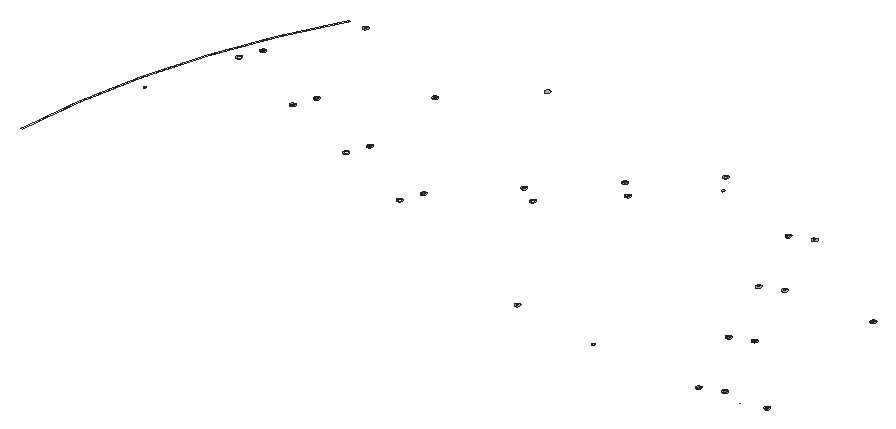
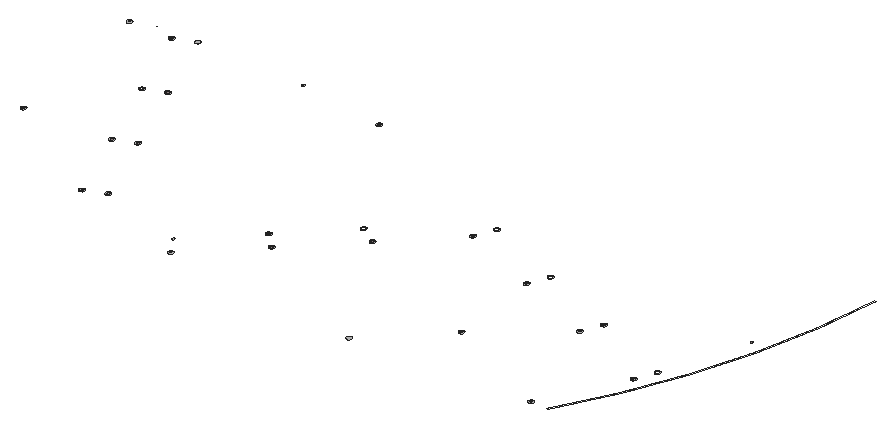
# SketchUp Ruby script. Lengths in inches.
U = 1.inch
M = Sketchup.active_model
def pt(a) = Geom::Point3d.new(a.map { |v| v * U })
def face(e, loops, mat)
  f = e.add_face(loops[0].map { |a| pt(a) })
  loops[1..].each { |l| e.add_face(l.map { |a| pt(a) }).erase! }
  f.material = f.back_material = mat if mat
  f
end
# faces: each face lists its corners as indices into pts; further lists are holes
def faces(e, pts, list, mat = nil) = list.each { |f| face(e, (f[0].is_a?(Array) ? f : [f]).map { |l| l.map { |i| pts[i] } }, mat) }
# xy, xz, yz: faces in a plane at the given z, y or x. An outline is a flat list of corners, or four numbers for a rectangle; further outlines are holes
def ring(l) = l.size == 4 ? [[l[0], l[1]], [l[2], l[1]], [l[2], l[3]], [l[0], l[3]]] : l.each_slice(2).to_a
def flat(e, list, mat, &to3) = list.each { |f| face(e, (f[0].is_a?(Array) ? f : [f]).map { |l| ring(l).map { |u, v| to3.(u, v) } }, mat) }
def xy(e, z, list, mat = nil) = flat(e, list, mat) { |x, y| [x, y, z] }
def xz(e, y, list, mat = nil) = flat(e, list, mat) { |x, z| [x, y, z] }
def yz(e, x, list, mat = nil) = flat(e, list, mat) { |y, z| [x, y, z] }
def lines(e, pts, list) = list.each { |a, b| e.add_line(pt(pts[a]), pt(pts[b])) }
# prism: a flat outline (further loops are holes) pulled along v
def prism(e, loops, v, mat = nil)
  f = face(e, loops, mat); d = Geom::Vector3d.new(v.map { |x| x * U })
  f.pushpull(f.normal.samedirection?(d) ? d.length : -d.length)
end
def box(e, o, s, mat = nil) = prism(e, [[o, [o[0] + s[0], o[1], o[2]], [o[0] + s[0], o[1] + s[1], o[2]], [o[0], o[1] + s[1], o[2]]]], [0, 0, s[2]], mat)
def at(x, y, z, deg = 0) = Geom::Transformation.translation(pt([x, y, z])) * Geom::Transformation.rotation(ORIGIN, Z_AXIS, deg.degrees)
def axes(o, x, y, z) = Geom::Transformation.new([*x, 0, *y, 0, *z, 0, *pt(o).to_a, 1])
def part(name) = M.definitions.add(name)
# library, detail: a bought-in or finely detailed component or shape, given as its bounding box
def library(name, o, s) = part(name).tap { |d| box(d.entities, o, s) }
def detail(e, o, s) = box(e.add_group.entities, o, s)
def put(e, d, t, mat = nil) = e.add_instance(d, t).tap { |i| i.material = mat if mat }
def group(e, t, mat = nil) = e.add_group.tap { |g| g.transformation = t; g.material = mat if mat }.entities
root = M.entities
M.materials.add("[Asphalt_Stamped_Brick]").color = [149, 133, 134]
M.materials.add("[Metal_Steel_Textured_White]").color = [191, 191, 191]
xy(root,3.625,[[149.02,166.314,149.015,166.316,149.011,166.32,149.008,166.324,149.006,166.329,149.005,166.334,149.006,166.339,149.008,166.344,149.011,166.348,149.015,166.351,149.02,166.353,149.025,166.354,149.031,166.353,149.035,166.351,149.04,166.348,149.043,166.344,149.045,166.339,149.045,166.329,149.043,166.324,149.04,166.32,149.035,166.316,149.031,166.314],[150.605,166.314,150.6,166.316,150.596,166.32,150.593,166.324,150.591,166.329,150.59,166.334,150.591,166.339,150.593,166.344,150.596,166.348,150.6,166.351,150.605,166.353,150.61,166.354,150.615,166.353,150.62,166.351,150.624,166.348,150.628,166.344,150.63,166.339,150.63,166.329,150.628,166.324,150.62,166.316,150.615,166.314],[141.054,166.555,141.049,166.556,141.044,166.558,141.04,166.561,141.037,166.565,141.035,166.57,141.034,166.575,141.035,166.581,141.037,166.585,141.04,166.59,141.044,166.593,141.049,166.595,141.059,166.595,141.064,166.593,141.068,166.59,141.071,166.585,141.073,166.581,141.074,166.575,141.073,166.57,141.071,166.565,141.068,166.561,141.064,166.558,141.059,166.556],[147.085,168.912,147.08,168.913,147.075,168.915,147.071,168.918,147.068,168.922,147.066,168.927,147.065,168.932,147.066,168.937,147.068,168.942,147.071,168.946,147.075,168.949,147.08,168.951,147.085,168.952,147.09,168.951,147.095,168.949,147.099,168.946,147.102,168.942,147.104,168.937,147.105,168.932,147.104,168.927,147.102,168.922,147.099,168.918,147.095,168.915,147.09,168.913],[124.428,169.885,124.423,169.886,124.418,169.888,124.414,169.891,124.411,169.895,124.409,169.9,124.408,169.905,124.409,169.91,124.411,169.915,124.414,169.919,124.418,169.922,124.423,169.924,124.428,169.925,124.433,169.924,124.438,169.922,124.442,169.919,124.446,169.915,124.448,169.91,124.448,169.9,124.446,169.895,124.442,169.891,124.438,169.888,124.433,169.886],
  [134.754,170.029,134.748,170.03,134.744,170.032,134.739,170.035,134.736,170.039,134.734,170.044,134.734,170.055,134.736,170.059,134.739,170.064,134.744,170.067,134.748,170.069,134.759,170.069,134.764,170.067,134.768,170.064,134.771,170.059,134.773,170.055,134.773,170.044,134.771,170.039,134.768,170.035,134.764,170.032,134.759,170.03],[131.754,171.272,131.748,171.273,131.744,171.275,131.739,171.278,131.736,171.282,131.734,171.287,131.734,171.297,131.736,171.302,131.739,171.306,131.744,171.309,131.748,171.311,131.754,171.312,131.759,171.311,131.764,171.309,131.768,171.306,131.771,171.302,131.773,171.297,131.774,171.292,131.773,171.287,131.771,171.282,131.768,171.278,131.764,171.275,131.759,171.273],[145.877,171.816,145.872,171.818,145.868,171.822,145.865,171.826,145.863,171.831,145.862,171.836,145.863,171.841,145.865,171.846,145.868,171.85,145.872,171.853,145.877,171.855,145.882,171.856,145.887,171.855,145.892,171.853,145.896,171.85,145.9,171.846,145.902,171.841,145.902,171.831,145.9,171.826,145.892,171.818,145.887,171.816],[146.62,172.121,146.615,172.122,146.61,172.124,146.606,172.127,146.603,172.131,146.601,172.136,146.6,172.141,146.601,172.146,146.603,172.151,146.606,172.155,146.61,172.159,146.615,172.161,146.625,172.161,146.63,172.159,146.634,172.155,146.637,172.151,146.639,172.146,146.64,172.141,146.639,172.136,146.637,172.131,146.634,172.127,146.63,172.124,146.625,172.122],[136.846,172.128,136.842,172.13,136.838,172.133,136.834,172.138,136.832,172.142,136.832,172.153,136.834,172.157,136.838,172.162,136.842,172.165,136.846,172.167,136.857,172.167,136.862,172.165,136.866,172.162,136.869,172.157,136.871,172.153,136.872,172.147,136.871,172.142,136.869,172.138,136.866,172.133,136.862,172.13,136.857,172.128],
  [128.748,172.515,128.744,172.517,128.736,172.525,128.734,172.529,128.734,172.54,128.736,172.545,128.74,172.549,128.744,172.552,128.748,172.554,128.754,172.555,128.759,172.554,128.764,172.552,128.768,172.549,128.771,172.545,128.773,172.54,128.774,172.535,128.773,172.529,128.771,172.525,128.768,172.521,128.764,172.517,128.759,172.515],[139.514,173.661,139.509,173.662,139.504,173.664,139.5,173.667,139.497,173.671,139.495,173.676,139.494,173.681,139.495,173.686,139.497,173.691,139.5,173.695,139.504,173.698,139.509,173.7,139.514,173.701,139.519,173.7,139.524,173.698,139.528,173.695,139.532,173.691,139.534,173.686,139.534,173.676,139.532,173.671,139.528,173.667,139.524,173.664,139.519,173.662],[125.754,173.757,125.749,173.758,125.744,173.76,125.74,173.763,125.736,173.767,125.734,173.772,125.734,173.782,125.736,173.787,125.744,173.795,125.749,173.797,125.759,173.797,125.764,173.795,125.768,173.791,125.771,173.787,125.773,173.782,125.774,173.777,125.773,173.772,125.771,173.767,125.768,173.763,125.764,173.76,125.759,173.758],[138.945,174.226,138.94,174.228,138.936,174.231,138.932,174.236,138.93,174.24,138.93,174.251,138.932,174.256,138.936,174.26,138.94,174.263,138.945,174.265,138.95,174.266,138.955,174.265,138.96,174.263,138.964,174.26,138.967,174.256,138.969,174.251,138.97,174.246,138.969,174.24,138.967,174.236,138.964,174.231,138.96,174.228,138.955,174.226],[131.439,174.713,131.434,174.714,131.429,174.716,131.425,174.719,131.422,174.723,131.42,174.728,131.419,174.733,131.42,174.738,131.422,174.743,131.425,174.747,131.429,174.75,131.434,174.752,131.439,174.753,131.444,174.752,131.449,174.75,131.453,174.747,131.456,174.743,131.458,174.738,131.459,174.733,131.458,174.728,131.456,174.723,131.453,174.719,131.449,174.716,131.444,174.714],
  [145.417,175.025,145.412,175.026,145.407,175.028,145.403,175.031,145.4,175.035,145.398,175.04,145.397,175.045,145.398,175.05,145.4,175.055,145.403,175.059,145.407,175.0625,145.412,175.064,145.417,175.065,145.422,175.064,145.427,175.0625,145.431,175.059,145.434,175.055,145.436,175.05,145.437,175.045,145.436,175.04,145.434,175.035,145.431,175.031,145.427,175.028,145.422,175.026],[127.249,176.695,127.244,176.696,127.239,176.698,127.235,176.701,127.232,176.705,127.23,176.71,127.229,176.715,127.23,176.72,127.232,176.725,127.235,176.729,127.239,176.732,127.244,176.734,127.249,176.735,127.254,176.734,127.259,176.732,127.263,176.729,127.266,176.725,127.268,176.72,127.269,176.715,127.268,176.71,127.266,176.705,127.263,176.701,127.259,176.698,127.254,176.696]],"[Asphalt_Stamped_Brick]")
xy(root,3.625,[[[148.288,165.939,148.265,165.942,148.243,165.951,148.225,165.965,148.211,165.984,148.202,166.005,148.199,166.028,148.202,166.051,148.211,166.073,148.225,166.091,148.243,166.105,148.265,166.114,148.288,166.117,148.311,166.114,148.332,166.105,148.351,166.091,148.365,166.073,148.374,166.051,148.377,166.028,148.374,166.005,148.365,165.984,148.351,165.965,148.332,165.951,148.311,165.942],[148.288,165.94,148.311,165.943,148.332,165.952,148.35,165.966,148.364,165.984,148.373,166.005,148.376,166.028,148.373,166.051,148.364,166.072,148.35,166.09,148.332,166.104,148.311,166.113,148.288,166.116,148.265,166.113,148.244,166.104,148.226,166.09,148.212,166.072,148.203,166.051,148.2,166.028,148.203,166.005,148.212,165.984,148.226,165.966,148.244,165.952,148.265,165.943]],[[148.288,165.94,148.265,165.943,148.244,165.952,148.226,165.966,148.212,165.984,148.203,166.005,148.2,166.028,148.203,166.051,148.212,166.072,148.226,166.09,148.244,166.104,148.265,166.113,148.288,166.116,148.311,166.113,148.332,166.104,148.35,166.09,148.364,166.072,148.373,166.051,148.376,166.028,148.373,166.005,148.364,165.984,148.35,165.966,148.332,165.952,148.311,165.943],[148.288,165.992,148.297,165.993,148.306,165.996,148.314,166.002,148.319,166.01,148.323,166.019,148.324,166.028,148.323,166.038,148.319,166.046,148.314,166.054,148.306,166.06,148.297,166.064,148.288,166.065,148.278,166.064,148.27,166.06,148.262,166.054,148.256,166.046,148.252,166.038,148.251,166.028,148.252,166.019,148.256,166.01,148.262,166.002,148.27,165.996,148.278,165.993]],[[144.263,166.074,144.254,166.075,144.245,166.079,144.237,166.084,144.232,166.092,144.228,166.101,144.227,166.11,144.228,166.12,144.232,166.129,144.237,166.136,144.245,166.142,144.254,166.146,144.263,166.147,144.273,166.146,144.282,166.142,144.289,166.136,144.295,166.129,144.299,166.12,144.3,166.11,144.299,166.101,144.295,166.092,144.289,166.084,144.282,166.079,144.273,166.075],[144.263,166.09,144.269,166.091,144.273,166.093,144.277,166.096,144.281,166.1,144.283,166.105,144.283,166.115,144.281,166.12,144.273,166.128,144.269,166.13,144.258,166.13,144.253,166.128,144.249,166.124,144.246,166.12,144.244,166.115,144.243,166.11,144.244,166.105,144.246,166.1,144.249,166.096,144.253,166.093,144.258,166.091]],[144.263,166.09,144.258,166.091,144.253,166.093,144.249,166.096,144.246,166.1,144.244,166.105,144.243,166.11,144.244,166.115,144.246,166.12,144.249,166.124,144.253,166.128,144.258,166.13,144.269,166.13,144.273,166.128,144.281,166.12,144.283,166.115,144.283,166.105,144.281,166.1,144.277,166.096,144.273,166.093,144.269,166.091],[[149.025,166.245,149.002,166.248,148.981,166.257,148.963,166.271,148.948,166.289,148.94,166.311,148.937,166.334,148.94,166.357,148.948,166.378,148.963,166.397,148.981,166.411,149.002,166.42,149.025,166.423,149.048,166.42,149.07,166.411,149.088,166.397,149.102,166.378,149.111,166.357,149.114,166.334,149.111,166.311,149.102,166.289,149.088,166.271,149.07,166.257,149.048,166.248],[149.025,166.246,149.048,166.249,149.069,166.258,149.088,166.272,149.102,166.29,149.11,166.311,149.113,166.334,149.11,166.356,149.102,166.378,149.088,166.396,149.069,166.41,149.048,166.419,149.025,166.422,149.003,166.419,148.981,166.41,148.963,166.396,148.949,166.378,148.941,166.356,148.9375,166.334,148.941,166.311,148.949,166.29,148.963,166.272,148.981,166.258,149.003,166.249]],
  [[149.025,166.246,149.003,166.249,148.981,166.258,148.963,166.272,148.949,166.29,148.941,166.311,148.9375,166.334,148.941,166.356,148.949,166.378,148.963,166.396,148.981,166.41,149.003,166.419,149.025,166.422,149.048,166.419,149.069,166.41,149.088,166.396,149.102,166.378,149.11,166.356,149.113,166.334,149.11,166.311,149.102,166.29,149.088,166.272,149.069,166.258,149.048,166.249],[149.025,166.297,149.035,166.298,149.044,166.302,149.051,166.308,149.057,166.315,149.061,166.324,149.062,166.334,149.061,166.343,149.057,166.352,149.051,166.36,149.044,166.365,149.035,166.369,149.025,166.37,149.016,166.369,149.007,166.365,149,166.36,148.994,166.352,148.99,166.343,148.989,166.334,148.99,166.324,148.994,166.315,149,166.308,149.007,166.302,149.016,166.298]],[[150.61,166.246,150.588,166.249,150.566,166.258,150.548,166.272,150.534,166.29,150.525,166.311,150.522,166.334,150.525,166.356,150.534,166.378,150.548,166.396,150.566,166.41,150.588,166.419,150.61,166.422,150.633,166.419,150.654,166.41,150.672,166.396,150.686,166.378,150.695,166.356,150.698,166.334,150.695,166.311,150.686,166.29,150.672,166.272,150.654,166.258,150.633,166.249],[150.61,166.297,150.62,166.298,150.629,166.302,150.636,166.308,150.642,166.315,150.646,166.324,150.647,166.334,150.646,166.343,150.642,166.352,150.636,166.36,150.629,166.365,150.62,166.369,150.61,166.37,150.601,166.369,150.592,166.365,150.584,166.36,150.579,166.352,150.575,166.343,150.574,166.334,150.575,166.324,150.579,166.315,150.584,166.308,150.592,166.302,150.601,166.298]],[[149.025,166.297,149.016,166.298,149.007,166.302,149,166.308,148.994,166.315,148.99,166.324,148.989,166.334,148.99,166.343,148.994,166.352,149,166.36,149.007,166.365,149.016,166.369,149.025,166.37,149.035,166.369,149.044,166.365,149.051,166.36,149.057,166.352,149.061,166.343,149.062,166.334,149.061,166.324,149.057,166.315,149.051,166.308,149.044,166.302,149.035,166.298],[149.02,166.314,149.031,166.314,149.035,166.316,149.04,166.32,149.043,166.324,149.045,166.329,149.045,166.339,149.043,166.344,149.04,166.348,149.035,166.351,149.031,166.353,149.025,166.354,149.02,166.353,149.015,166.351,149.011,166.348,149.008,166.344,149.006,166.339,149.005,166.334,149.006,166.329,149.008,166.324,149.011,166.32,149.015,166.316]],[[150.61,166.297,150.601,166.298,150.592,166.302,150.584,166.308,150.579,166.315,150.575,166.324,150.574,166.334,150.575,166.343,150.579,166.352,150.584,166.36,150.592,166.365,150.601,166.369,150.61,166.37,150.62,166.369,150.629,166.365,150.636,166.36,150.642,166.352,150.646,166.343,150.647,166.334,150.646,166.324,150.642,166.315,150.636,166.308,150.629,166.302,150.62,166.298],[150.605,166.314,150.615,166.314,150.62,166.316,150.628,166.324,150.63,166.329,150.63,166.339,150.628,166.344,150.624,166.348,150.62,166.351,150.615,166.353,150.61,166.354,150.605,166.353,150.6,166.351,150.596,166.348,150.593,166.344,150.591,166.339,150.59,166.334,150.591,166.329,150.593,166.324,150.596,166.32,150.6,166.316]],[[141.054,166.488,141.031,166.491,141.01,166.499,140.992,166.513,140.978,166.531,140.969,166.553,140.966,166.575,140.969,166.598,140.978,166.619,140.992,166.638,141.01,166.652,141.031,166.66,141.054,166.663,141.077,166.66,141.098,166.652,141.116,166.638,141.13,166.619,141.139,166.598,141.142,166.575,141.139,166.553,141.13,166.531,141.116,166.513,141.098,166.499,141.077,166.491],[141.054,166.539,141.063,166.54,141.072,166.544,141.08,166.55,141.086,166.557,141.089,166.566,141.091,166.575,141.089,166.585,141.086,166.594,141.08,166.601,141.072,166.607,141.063,166.611,141.054,166.612,141.045,166.611,141.036,166.607,141.028,166.601,141.022,166.594,141.019,166.585,141.017,166.575,141.019,166.566,141.022,166.557,141.028,166.55,141.036,166.544,141.045,166.54]],
  [[141.054,166.539,141.045,166.54,141.036,166.544,141.028,166.55,141.022,166.557,141.019,166.566,141.017,166.575,141.019,166.585,141.022,166.594,141.028,166.601,141.036,166.607,141.045,166.611,141.054,166.612,141.063,166.611,141.072,166.607,141.08,166.601,141.086,166.594,141.089,166.585,141.091,166.575,141.089,166.566,141.086,166.557,141.08,166.55,141.072,166.544,141.063,166.54],[141.054,166.555,141.059,166.556,141.064,166.558,141.068,166.561,141.071,166.565,141.073,166.57,141.074,166.575,141.073,166.581,141.071,166.585,141.068,166.59,141.064,166.593,141.059,166.595,141.049,166.595,141.044,166.593,141.04,166.59,141.037,166.585,141.035,166.581,141.034,166.575,141.035,166.57,141.037,166.565,141.04,166.561,141.044,166.558,141.049,166.556]],[[147.085,168.843,147.062,168.846,147.041,168.855,147.022,168.869,147.008,168.888,146.999,168.909,146.996,168.932,146.999,168.955,147.008,168.976,147.022,168.995,147.041,169.009,147.062,169.018,147.085,169.021,147.108,169.018,147.129,169.009,147.148,168.995,147.162,168.976,147.171,168.955,147.174,168.932,147.171,168.909,147.162,168.888,147.148,168.869,147.129,168.855,147.108,168.846],[147.085,168.844,147.108,168.847,147.129,168.856,147.147,168.87,147.161,168.888,147.17,168.909,147.173,168.932,147.17,168.955,147.161,168.976,147.147,168.994,147.129,169.008,147.108,169.017,147.085,169.02,147.062,169.017,147.041,169.008,147.023,168.994,147.009,168.976,147,168.955,146.997,168.932,147,168.909,147.009,168.888,147.023,168.87,147.041,168.856,147.062,168.847]],[[147.085,168.844,147.062,168.847,147.041,168.856,147.023,168.87,147.009,168.888,147,168.909,146.997,168.932,147,168.955,147.009,168.976,147.023,168.994,147.041,169.008,147.062,169.017,147.085,169.02,147.108,169.017,147.129,169.008,147.147,168.994,147.161,168.976,147.17,168.955,147.173,168.932,147.17,168.909,147.161,168.888,147.147,168.87,147.129,168.856,147.108,168.847],[147.085,168.895,147.094,168.897,147.103,168.9,147.111,168.906,147.117,168.914,147.12,168.923,147.122,168.932,147.12,168.941,147.117,168.95,147.111,168.958,147.103,168.964,147.094,168.967,147.085,168.969,147.076,168.967,147.067,168.964,147.059,168.958,147.053,168.95,147.05,168.941,147.048,168.932,147.05,168.923,147.053,168.914,147.059,168.906,147.067,168.9,147.076,168.897]],[[147.085,168.895,147.076,168.897,147.067,168.9,147.059,168.906,147.053,168.914,147.05,168.923,147.048,168.932,147.05,168.941,147.053,168.95,147.059,168.958,147.067,168.964,147.076,168.967,147.085,168.969,147.094,168.967,147.103,168.964,147.111,168.958,147.117,168.95,147.12,168.941,147.122,168.932,147.12,168.923,147.117,168.914,147.111,168.906,147.103,168.9,147.094,168.897],[147.085,168.912,147.09,168.913,147.095,168.915,147.099,168.918,147.102,168.922,147.104,168.927,147.105,168.932,147.104,168.937,147.102,168.942,147.099,168.946,147.095,168.949,147.09,168.951,147.085,168.952,147.08,168.951,147.075,168.949,147.071,168.946,147.068,168.942,147.066,168.937,147.065,168.932,147.066,168.927,147.068,168.922,147.071,168.918,147.075,168.915,147.08,168.913]],[[147.823,169.149,147.8,169.152,147.778,169.161,147.76,169.175,147.746,169.193,147.737,169.215,147.734,169.238,147.737,169.261,147.746,169.282,147.76,169.3,147.778,169.315,147.8,169.323,147.823,169.326,147.846,169.323,147.867,169.315,147.886,169.3,147.9,169.282,147.909,169.261,147.912,169.238,147.909,169.215,147.9,169.193,147.886,169.175,147.867,169.161,147.846,169.152],[147.823,169.15,147.845,169.153,147.867,169.161,147.885,169.175,147.899,169.194,147.908,169.215,147.911,169.238,147.908,169.26,147.899,169.281,147.885,169.3,147.867,169.314,147.845,169.322,147.823,169.325,147.8,169.322,147.779,169.314,147.76,169.3,147.747,169.281,147.738,169.26,147.735,169.238,147.738,169.215,147.747,169.194,147.76,169.175,147.779,169.161,147.8,169.153]],
  [[134.448,169.223,134.425,169.226,134.404,169.235,134.385,169.249,134.371,169.267,134.362,169.289,134.359,169.312,134.362,169.335,134.371,169.356,134.385,169.375,134.404,169.389,134.425,169.398,134.448,169.401,134.471,169.398,134.492,169.389,134.511,169.375,134.525,169.356,134.534,169.335,134.537,169.312,134.534,169.289,134.525,169.267,134.511,169.249,134.492,169.235,134.471,169.226],[134.448,169.224,134.471,169.227,134.492,169.236,134.51,169.25,134.524,169.268,134.533,169.289,134.536,169.312,134.533,169.334,134.524,169.356,134.51,169.374,134.492,169.388,134.471,169.397,134.448,169.4,134.425,169.397,134.404,169.388,134.386,169.374,134.372,169.356,134.363,169.334,134.36,169.312,134.363,169.289,134.372,169.268,134.386,169.25,134.404,169.236,134.425,169.227]],[[124.428,169.868,124.419,169.87,124.41,169.873,124.402,169.879,124.397,169.887,124.393,169.896,124.392,169.905,124.393,169.914,124.397,169.923,124.402,169.931,124.41,169.937,124.419,169.94,124.428,169.942,124.438,169.94,124.447,169.937,124.454,169.931,124.46,169.923,124.464,169.914,124.465,169.905,124.464,169.896,124.46,169.887,124.454,169.879,124.447,169.873,124.438,169.87],[124.428,169.885,124.433,169.886,124.438,169.888,124.442,169.891,124.446,169.895,124.448,169.9,124.448,169.91,124.446,169.915,124.442,169.919,124.438,169.922,124.433,169.924,124.428,169.925,124.423,169.924,124.418,169.922,124.414,169.919,124.411,169.915,124.409,169.91,124.408,169.905,124.409,169.9,124.411,169.895,124.414,169.891,124.418,169.888,124.423,169.886]],[[134.754,169.961,134.731,169.964,134.709,169.972,134.691,169.987,134.677,170.005,134.668,170.026,134.665,170.049,134.668,170.072,134.677,170.094,134.691,170.112,134.709,170.126,134.731,170.135,134.754,170.138,134.777,170.135,134.798,170.126,134.816,170.112,134.831,170.094,134.839,170.072,134.842,170.049,134.839,170.026,134.831,170.005,134.816,169.987,134.798,169.972,134.777,169.964],[134.754,169.961,134.776,169.964,134.798,169.973,134.816,169.987,134.83,170.005,134.838,170.027,134.841,170.049,134.838,170.072,134.83,170.093,134.816,170.112,134.798,170.126,134.776,170.134,134.754,170.137,134.731,170.134,134.71,170.126,134.691,170.112,134.677,170.093,134.669,170.072,134.666,170.049,134.669,170.027,134.677,170.005,134.691,169.987,134.71,169.973,134.731,169.964]],[[134.754,169.961,134.731,169.964,134.71,169.973,134.691,169.987,134.677,170.005,134.669,170.027,134.666,170.049,134.669,170.072,134.677,170.093,134.691,170.112,134.71,170.126,134.731,170.134,134.754,170.137,134.776,170.134,134.798,170.126,134.816,170.112,134.83,170.093,134.838,170.072,134.841,170.049,134.838,170.027,134.83,170.005,134.816,169.987,134.798,169.973,134.776,169.964],[134.754,170.013,134.763,170.014,134.772,170.018,134.779,170.024,134.785,170.031,134.789,170.04,134.79,170.049,134.789,170.059,134.785,170.068,134.779,170.075,134.772,170.081,134.763,170.085,134.754,170.086,134.744,170.085,134.735,170.081,134.728,170.075,134.722,170.068,134.718,170.059,134.717,170.049,134.718,170.04,134.722,170.031,134.728,170.024,134.735,170.018,134.744,170.014]],[[134.754,170.013,134.744,170.014,134.735,170.018,134.728,170.024,134.722,170.031,134.718,170.04,134.717,170.049,134.718,170.059,134.722,170.068,134.728,170.075,134.735,170.081,134.744,170.085,134.754,170.086,134.763,170.085,134.772,170.081,134.779,170.075,134.785,170.068,134.789,170.059,134.79,170.049,134.789,170.04,134.785,170.031,134.779,170.024,134.772,170.018,134.763,170.014],[134.754,170.029,134.759,170.03,134.764,170.032,134.768,170.035,134.771,170.039,134.773,170.044,134.773,170.055,134.771,170.059,134.768,170.064,134.764,170.067,134.759,170.069,134.748,170.069,134.744,170.067,134.739,170.064,134.736,170.059,134.734,170.055,134.734,170.044,134.736,170.039,134.739,170.035,134.744,170.032,134.748,170.03]],
  [[131.448,170.465,131.425,170.468,131.404,170.477,131.385,170.492,131.371,170.51,131.362,170.531,131.359,170.554,131.362,170.577,131.371,170.599,131.385,170.617,131.404,170.631,131.425,170.64,131.448,170.643,131.471,170.64,131.492,170.631,131.511,170.617,131.525,170.599,131.534,170.577,131.537,170.554,131.534,170.531,131.525,170.51,131.511,170.492,131.492,170.477,131.471,170.468],[131.448,170.466,131.471,170.469,131.492,170.478,131.51,170.492,131.524,170.51,131.533,170.532,131.536,170.554,131.533,170.577,131.524,170.598,131.51,170.617,131.492,170.631,131.471,170.639,131.448,170.642,131.425,170.639,131.404,170.631,131.386,170.617,131.372,170.598,131.363,170.577,131.36,170.554,131.363,170.532,131.372,170.51,131.386,170.492,131.404,170.478,131.425,170.469]],[[131.754,171.203,131.731,171.206,131.709,171.215,131.691,171.229,131.677,171.248,131.668,171.269,131.665,171.292,131.668,171.315,131.677,171.336,131.691,171.355,131.709,171.369,131.731,171.378,131.754,171.381,131.777,171.378,131.798,171.369,131.816,171.355,131.831,171.336,131.839,171.315,131.842,171.292,131.839,171.269,131.831,171.248,131.816,171.229,131.798,171.215,131.777,171.206],[131.754,171.204,131.776,171.207,131.798,171.216,131.816,171.23,131.83,171.248,131.839,171.269,131.842,171.292,131.839,171.315,131.83,171.336,131.816,171.354,131.798,171.368,131.776,171.377,131.754,171.38,131.731,171.377,131.71,171.368,131.691,171.354,131.677,171.336,131.669,171.315,131.666,171.292,131.669,171.269,131.677,171.248,131.691,171.23,131.71,171.216,131.731,171.207]],[[131.754,171.204,131.731,171.207,131.71,171.216,131.691,171.23,131.677,171.248,131.669,171.269,131.666,171.292,131.669,171.315,131.677,171.336,131.691,171.354,131.71,171.368,131.731,171.377,131.754,171.38,131.776,171.377,131.798,171.368,131.816,171.354,131.83,171.336,131.839,171.315,131.842,171.292,131.839,171.269,131.83,171.248,131.816,171.23,131.798,171.216,131.776,171.207],[131.754,171.255,131.763,171.257,131.772,171.26,131.779,171.266,131.785,171.274,131.789,171.283,131.79,171.292,131.789,171.301,131.785,171.31,131.779,171.318,131.772,171.324,131.763,171.327,131.754,171.329,131.744,171.327,131.735,171.324,131.728,171.318,131.722,171.31,131.718,171.301,131.717,171.292,131.718,171.283,131.722,171.274,131.728,171.266,131.735,171.26,131.744,171.257]],[[131.754,171.255,131.744,171.257,131.735,171.26,131.728,171.266,131.722,171.274,131.718,171.283,131.717,171.292,131.718,171.301,131.722,171.31,131.728,171.318,131.735,171.324,131.744,171.327,131.754,171.329,131.763,171.327,131.772,171.324,131.779,171.318,131.785,171.31,131.789,171.301,131.79,171.292,131.789,171.283,131.785,171.274,131.779,171.266,131.772,171.26,131.763,171.257],[131.754,171.272,131.759,171.273,131.764,171.275,131.768,171.278,131.771,171.282,131.773,171.287,131.774,171.292,131.773,171.297,131.771,171.302,131.768,171.306,131.764,171.309,131.759,171.311,131.754,171.312,131.748,171.311,131.744,171.309,131.739,171.306,131.736,171.302,131.734,171.297,131.734,171.287,131.736,171.282,131.739,171.278,131.744,171.275,131.748,171.273]],[[137.533,171.611,137.51,171.614,137.489,171.623,137.47,171.637,137.456,171.655,137.447,171.677,137.444,171.7,137.447,171.723,137.456,171.744,137.47,171.763,137.489,171.777,137.51,171.786,137.533,171.789,137.556,171.786,137.578,171.777,137.596,171.763,137.61,171.744,137.619,171.723,137.622,171.7,137.619,171.677,137.61,171.655,137.596,171.637,137.578,171.623,137.556,171.614],[137.533,171.612,137.556,171.615,137.577,171.624,137.595,171.638,137.609,171.656,137.618,171.677,137.621,171.7,137.618,171.723,137.609,171.744,137.595,171.762,137.577,171.776,137.556,171.785,137.533,171.788,137.51,171.785,137.489,171.776,137.471,171.762,137.457,171.744,137.448,171.723,137.445,171.7,137.448,171.677,137.457,171.656,137.471,171.638,137.489,171.624,137.51,171.615]],
  [[128.448,171.708,128.425,171.711,128.404,171.72,128.385,171.734,128.371,171.753,128.362,171.774,128.359,171.797,128.362,171.82,128.371,171.841,128.385,171.86,128.404,171.874,128.425,171.883,128.448,171.886,128.471,171.883,128.493,171.874,128.511,171.86,128.525,171.841,128.534,171.82,128.537,171.797,128.534,171.774,128.525,171.753,128.511,171.734,128.493,171.72,128.471,171.711],[128.448,171.709,128.471,171.712,128.492,171.721,128.51,171.735,128.524,171.753,128.533,171.774,128.536,171.797,128.533,171.82,128.524,171.841,128.51,171.859,128.492,171.873,128.471,171.882,128.448,171.885,128.425,171.882,128.404,171.873,128.386,171.859,128.372,171.841,128.363,171.82,128.36,171.797,128.363,171.774,128.372,171.753,128.386,171.735,128.404,171.721,128.425,171.712]],[[145.882,171.748,145.859,171.751,145.838,171.76,145.82,171.774,145.806,171.792,145.797,171.813,145.794,171.836,145.797,171.859,145.806,171.88,145.82,171.898,145.838,171.912,145.859,171.921,145.882,171.924,145.905,171.921,145.926,171.912,145.944,171.898,145.958,171.88,145.967,171.859,145.97,171.836,145.967,171.813,145.958,171.792,145.944,171.774,145.926,171.76,145.905,171.751],[145.882,171.799,145.892,171.8,145.901,171.804,145.908,171.81,145.914,171.817,145.918,171.826,145.919,171.836,145.918,171.845,145.914,171.854,145.908,171.862,145.901,171.867,145.892,171.871,145.882,171.872,145.873,171.871,145.864,171.867,145.856,171.862,145.851,171.854,145.847,171.845,145.846,171.836,145.847,171.826,145.851,171.817,145.856,171.81,145.864,171.804,145.873,171.8]],[[145.882,171.799,145.873,171.8,145.864,171.804,145.856,171.81,145.851,171.817,145.847,171.826,145.846,171.836,145.847,171.845,145.851,171.854,145.856,171.862,145.864,171.867,145.873,171.871,145.882,171.872,145.892,171.871,145.901,171.867,145.908,171.862,145.914,171.854,145.918,171.845,145.919,171.836,145.918,171.826,145.914,171.817,145.908,171.81,145.901,171.804,145.892,171.8],[145.877,171.816,145.887,171.816,145.892,171.818,145.9,171.826,145.902,171.831,145.902,171.841,145.9,171.846,145.896,171.85,145.892,171.853,145.887,171.855,145.882,171.856,145.877,171.855,145.872,171.853,145.868,171.85,145.865,171.846,145.863,171.841,145.862,171.836,145.863,171.831,145.865,171.826,145.868,171.822,145.872,171.818]],[[146.62,172.053,146.597,172.056,146.576,172.065,146.558,172.079,146.544,172.097,146.535,172.119,146.532,172.141,146.535,172.164,146.544,172.185,146.558,172.203,146.576,172.217,146.597,172.226,146.62,172.229,146.643,172.226,146.664,172.217,146.682,172.203,146.696,172.185,146.705,172.164,146.708,172.141,146.705,172.119,146.696,172.097,146.682,172.079,146.664,172.065,146.643,172.056],[146.62,172.105,146.629,172.106,146.638,172.11,146.646,172.115,146.652,172.123,146.655,172.132,146.656,172.141,146.655,172.151,146.652,172.16,146.646,172.167,146.638,172.173,146.629,172.177,146.62,172.178,146.61,172.177,146.602,172.173,146.594,172.167,146.588,172.16,146.585,172.151,146.583,172.141,146.585,172.132,146.588,172.123,146.594,172.115,146.602,172.11,146.61,172.106]],[[136.852,172.06,136.829,172.0625,136.808,172.071,136.789,172.085,136.775,172.104,136.767,172.125,136.764,172.147,136.767,172.17,136.775,172.191,136.789,172.21,136.808,172.224,136.829,172.232,136.852,172.235,136.874,172.232,136.896,172.224,136.914,172.21,136.928,172.191,136.937,172.17,136.94,172.147,136.937,172.125,136.928,172.104,136.914,172.085,136.896,172.071,136.874,172.0625],[136.852,172.111,136.861,172.112,136.87,172.116,136.878,172.122,136.883,172.129,136.887,172.138,136.888,172.147,136.887,172.157,136.883,172.166,136.878,172.173,136.87,172.179,136.861,172.183,136.852,172.184,136.842,172.183,136.833,172.179,136.826,172.173,136.82,172.166,136.816,172.157,136.815,172.147,136.816,172.138,136.82,172.129,136.826,172.122,136.833,172.116,136.842,172.112]],
  [[146.62,172.105,146.61,172.106,146.602,172.11,146.594,172.115,146.588,172.123,146.585,172.132,146.583,172.141,146.585,172.151,146.588,172.16,146.594,172.167,146.602,172.173,146.61,172.177,146.62,172.178,146.629,172.177,146.638,172.173,146.646,172.167,146.652,172.16,146.655,172.151,146.656,172.141,146.655,172.132,146.652,172.123,146.646,172.115,146.638,172.11,146.629,172.106],[146.62,172.121,146.625,172.122,146.63,172.124,146.634,172.127,146.637,172.131,146.639,172.136,146.64,172.141,146.639,172.146,146.637,172.151,146.634,172.155,146.63,172.159,146.625,172.161,146.615,172.161,146.61,172.159,146.606,172.155,146.603,172.151,146.601,172.146,146.6,172.141,146.601,172.136,146.603,172.131,146.606,172.127,146.61,172.124,146.615,172.122]],[[136.852,172.111,136.842,172.112,136.833,172.116,136.826,172.122,136.82,172.129,136.816,172.138,136.815,172.147,136.816,172.157,136.82,172.166,136.826,172.173,136.833,172.179,136.842,172.183,136.852,172.184,136.861,172.183,136.87,172.179,136.878,172.173,136.883,172.166,136.887,172.157,136.888,172.147,136.887,172.138,136.883,172.129,136.878,172.122,136.87,172.116,136.861,172.112],[136.846,172.128,136.857,172.128,136.862,172.13,136.866,172.133,136.869,172.138,136.871,172.142,136.872,172.147,136.871,172.153,136.869,172.157,136.866,172.162,136.862,172.165,136.857,172.167,136.846,172.167,136.842,172.165,136.838,172.162,136.834,172.157,136.832,172.153,136.832,172.142,136.834,172.138,136.838,172.133,136.842,172.13]],[149.818,172.204,149.795,172.207,149.773,172.216,149.755,172.23,149.741,172.249,149.732,172.27,149.729,172.293,149.732,172.316,149.741,172.338,149.755,172.356,149.773,172.37,149.795,172.379,149.818,172.382,149.818,172.381,149.795,172.378,149.774,172.369,149.756,172.355,149.742,172.337,149.733,172.316,149.73,172.293,149.733,172.271,149.742,172.249,149.756,172.231,149.774,172.217,149.795,172.208,149.818,172.205],[[149.818,172.204,149.818,172.205,149.795,172.208,149.774,172.217,149.756,172.231,149.742,172.249,149.733,172.271,149.73,172.293,149.733,172.316,149.742,172.337,149.756,172.355,149.774,172.369,149.795,172.378,149.818,172.381,149.818,172.382,149.841,172.379,149.862,172.37,149.881,172.356,149.895,172.338,149.904,172.316,149.907,172.293,149.904,172.27,149.895,172.249,149.881,172.23,149.862,172.216,149.841,172.207],[149.818,172.273,149.818,172.313,149.813,172.3125,149.808,172.311,149.804,172.307,149.801,172.303,149.799,172.298,149.798,172.293,149.799,172.288,149.801,172.283,149.804,172.279,149.808,172.276,149.813,172.274]],[149.818,172.205,149.818,172.273,149.823,172.274,149.828,172.276,149.832,172.279,149.835,172.283,149.837,172.288,149.838,172.293,149.837,172.298,149.835,172.303,149.832,172.307,149.828,172.311,149.823,172.3125,149.818,172.313,149.818,172.381,149.841,172.378,149.862,172.369,149.88,172.355,149.894,172.337,149.903,172.316,149.906,172.293,149.903,172.271,149.894,172.249,149.88,172.231,149.862,172.217,149.841,172.208],
  [149.818,172.273,149.813,172.274,149.808,172.276,149.804,172.279,149.801,172.283,149.799,172.288,149.798,172.293,149.799,172.298,149.801,172.303,149.804,172.307,149.808,172.311,149.813,172.3125,149.818,172.313],[[128.754,172.446,128.731,172.449,128.709,172.458,128.691,172.472,128.677,172.49,128.668,172.512,128.665,172.535,128.668,172.558,128.677,172.579,128.691,172.597,128.709,172.612,128.731,172.62,128.754,172.624,128.777,172.62,128.798,172.612,128.816,172.597,128.831,172.579,128.839,172.558,128.843,172.535,128.839,172.512,128.831,172.49,128.816,172.472,128.798,172.458,128.777,172.449],[128.754,172.447,128.776,172.45,128.798,172.458,128.816,172.472,128.83,172.491,128.839,172.512,128.842,172.535,128.839,172.557,128.83,172.579,128.816,172.597,128.798,172.611,128.776,172.62,128.754,172.623,128.731,172.62,128.71,172.611,128.691,172.597,128.677,172.579,128.669,172.557,128.666,172.535,128.669,172.512,128.677,172.491,128.691,172.472,128.71,172.458,128.731,172.45]],[[128.754,172.447,128.731,172.45,128.71,172.458,128.691,172.472,128.677,172.491,128.669,172.512,128.666,172.535,128.669,172.557,128.677,172.579,128.691,172.597,128.71,172.611,128.731,172.62,128.754,172.623,128.776,172.62,128.798,172.611,128.816,172.597,128.83,172.579,128.839,172.557,128.842,172.535,128.839,172.512,128.83,172.491,128.816,172.472,128.798,172.458,128.776,172.45],[128.754,172.498,128.763,172.499,128.772,172.503,128.78,172.509,128.785,172.516,128.789,172.525,128.79,172.535,128.789,172.544,128.785,172.553,128.78,172.561,128.772,172.566,128.763,172.57,128.754,172.571,128.744,172.57,128.735,172.566,128.728,172.561,128.722,172.553,128.718,172.544,128.717,172.535,128.718,172.525,128.722,172.516,128.728,172.509,128.735,172.503,128.744,172.499]],[[128.754,172.498,128.744,172.499,128.735,172.503,128.728,172.509,128.722,172.516,128.718,172.525,128.717,172.535,128.718,172.544,128.722,172.553,128.728,172.561,128.735,172.566,128.744,172.57,128.754,172.571,128.763,172.57,128.772,172.566,128.78,172.561,128.785,172.553,128.789,172.544,128.79,172.535,128.789,172.525,128.785,172.516,128.78,172.509,128.772,172.503,128.763,172.499],[128.748,172.515,128.759,172.515,128.764,172.517,128.768,172.521,128.771,172.525,128.773,172.529,128.774,172.535,128.773,172.54,128.771,172.545,128.768,172.549,128.764,172.552,128.759,172.554,128.754,172.555,128.748,172.554,128.744,172.552,128.74,172.549,128.736,172.545,128.734,172.54,128.734,172.529,128.736,172.525,128.744,172.517]],[[125.448,172.951,125.425,172.954,125.404,172.963,125.385,172.977,125.371,172.995,125.362,173.017,125.359,173.04,125.362,173.0625,125.371,173.084,125.385,173.102,125.404,173.117,125.425,173.125,125.448,173.128,125.471,173.125,125.493,173.117,125.511,173.102,125.525,173.084,125.534,173.0625,125.537,173.04,125.534,173.017,125.525,172.995,125.511,172.977,125.493,172.963,125.471,172.954],[125.448,172.952,125.471,172.955,125.492,172.963,125.51,172.977,125.524,172.996,125.533,173.017,125.536,173.04,125.533,173.0625,125.524,173.084,125.51,173.102,125.492,173.116,125.471,173.125,125.448,173.128,125.425,173.125,125.404,173.116,125.386,173.102,125.372,173.084,125.363,173.0625,125.36,173.04,125.363,173.017,125.372,172.996,125.386,172.977,125.404,172.963,125.425,172.955]],
  [[139.514,173.592,139.491,173.595,139.47,173.604,139.451,173.618,139.4375,173.637,139.428,173.658,139.425,173.681,139.428,173.704,139.4375,173.725,139.451,173.744,139.47,173.758,139.491,173.767,139.514,173.77,139.537,173.767,139.559,173.758,139.577,173.744,139.591,173.725,139.6,173.704,139.603,173.681,139.6,173.658,139.591,173.637,139.577,173.618,139.559,173.604,139.537,173.595],[139.514,173.593,139.537,173.596,139.558,173.605,139.576,173.619,139.59,173.637,139.599,173.658,139.602,173.681,139.599,173.704,139.59,173.725,139.576,173.743,139.558,173.757,139.537,173.766,139.514,173.769,139.492,173.766,139.47,173.757,139.452,173.743,139.438,173.725,139.429,173.704,139.426,173.681,139.429,173.658,139.438,173.637,139.452,173.619,139.47,173.605,139.492,173.596]],[[139.514,173.593,139.492,173.596,139.47,173.605,139.452,173.619,139.438,173.637,139.429,173.658,139.426,173.681,139.429,173.704,139.438,173.725,139.452,173.743,139.47,173.757,139.492,173.766,139.514,173.769,139.537,173.766,139.558,173.757,139.576,173.743,139.59,173.725,139.599,173.704,139.602,173.681,139.599,173.658,139.59,173.637,139.576,173.619,139.558,173.605,139.537,173.596],[139.514,173.644,139.524,173.646,139.533,173.649,139.54,173.655,139.546,173.663,139.55,173.672,139.551,173.681,139.55,173.69,139.546,173.699,139.54,173.707,139.533,173.713,139.524,173.716,139.514,173.718,139.505,173.716,139.496,173.713,139.488,173.707,139.483,173.699,139.479,173.69,139.478,173.681,139.479,173.672,139.483,173.663,139.488,173.655,139.496,173.649,139.505,173.646]],[[139.514,173.644,139.505,173.646,139.496,173.649,139.488,173.655,139.483,173.663,139.479,173.672,139.478,173.681,139.479,173.69,139.483,173.699,139.488,173.707,139.496,173.713,139.505,173.716,139.514,173.718,139.524,173.716,139.533,173.713,139.54,173.707,139.546,173.699,139.55,173.69,139.551,173.681,139.55,173.672,139.546,173.663,139.54,173.655,139.533,173.649,139.524,173.646],[139.514,173.661,139.519,173.662,139.524,173.664,139.528,173.667,139.532,173.671,139.534,173.676,139.534,173.686,139.532,173.691,139.528,173.695,139.524,173.698,139.519,173.7,139.514,173.701,139.509,173.7,139.504,173.698,139.5,173.695,139.497,173.691,139.495,173.686,139.494,173.681,139.495,173.676,139.497,173.671,139.5,173.667,139.504,173.664,139.509,173.662]],[[125.754,173.688,125.731,173.691,125.709,173.7,125.691,173.714,125.677,173.733,125.668,173.754,125.665,173.777,125.668,173.8,125.677,173.822,125.691,173.84,125.709,173.854,125.731,173.863,125.754,173.866,125.777,173.863,125.798,173.854,125.817,173.84,125.831,173.822,125.84,173.8,125.843,173.777,125.84,173.754,125.831,173.733,125.817,173.714,125.798,173.7,125.777,173.691],[125.754,173.689,125.776,173.692,125.798,173.701,125.816,173.715,125.83,173.733,125.839,173.755,125.842,173.777,125.839,173.8,125.83,173.821,125.816,173.839,125.798,173.853,125.776,173.862,125.754,173.865,125.731,173.862,125.71,173.853,125.691,173.839,125.678,173.821,125.669,173.8,125.666,173.777,125.669,173.755,125.678,173.733,125.691,173.715,125.71,173.701,125.731,173.692]],[[125.754,173.741,125.744,173.742,125.735,173.746,125.728,173.751,125.722,173.759,125.718,173.768,125.717,173.777,125.718,173.787,125.722,173.796,125.728,173.803,125.735,173.809,125.744,173.8125,125.754,173.814,125.763,173.8125,125.772,173.809,125.78,173.803,125.785,173.796,125.789,173.787,125.79,173.777,125.789,173.768,125.785,173.759,125.78,173.751,125.772,173.746,125.763,173.742],[125.754,173.757,125.759,173.758,125.764,173.76,125.768,173.763,125.771,173.767,125.773,173.772,125.774,173.777,125.773,173.782,125.771,173.787,125.768,173.791,125.764,173.795,125.759,173.797,125.749,173.797,125.744,173.795,125.736,173.787,125.734,173.782,125.734,173.772,125.736,173.767,125.74,173.763,125.744,173.76,125.749,173.758]],
  [[138.95,174.157,138.927,174.16,138.905,174.169,138.887,174.183,138.873,174.201,138.864,174.223,138.861,174.246,138.864,174.269,138.873,174.29,138.887,174.308,138.905,174.323,138.927,174.331,138.95,174.334,138.973,174.331,138.994,174.323,139.013,174.308,139.027,174.29,139.036,174.269,139.039,174.246,139.036,174.223,139.027,174.201,139.013,174.183,138.994,174.169,138.973,174.16],[138.95,174.158,138.972,174.161,138.994,174.169,139.012,174.183,139.026,174.202,139.035,174.223,139.038,174.246,139.035,174.268,139.026,174.29,139.012,174.308,138.994,174.322,138.972,174.331,138.95,174.334,138.927,174.331,138.906,174.322,138.888,174.308,138.874,174.29,138.865,174.268,138.862,174.246,138.865,174.223,138.874,174.202,138.888,174.183,138.906,174.169,138.927,174.161]],[[138.95,174.158,138.927,174.161,138.906,174.169,138.888,174.183,138.874,174.202,138.865,174.223,138.862,174.246,138.865,174.268,138.874,174.29,138.888,174.308,138.906,174.322,138.927,174.331,138.95,174.334,138.972,174.331,138.994,174.322,139.012,174.308,139.026,174.29,139.035,174.268,139.038,174.246,139.035,174.223,139.026,174.202,139.012,174.183,138.994,174.169,138.972,174.161],[138.95,174.209,138.959,174.21,138.968,174.214,138.976,174.22,138.981,174.227,138.985,174.236,138.986,174.246,138.985,174.255,138.981,174.264,138.976,174.271,138.968,174.277,138.959,174.281,138.95,174.282,138.94,174.281,138.931,174.277,138.924,174.271,138.918,174.264,138.914,174.255,138.913,174.246,138.914,174.236,138.918,174.227,138.924,174.22,138.931,174.214,138.94,174.21]],[[138.95,174.209,138.94,174.21,138.931,174.214,138.924,174.22,138.918,174.227,138.914,174.236,138.913,174.246,138.914,174.255,138.918,174.264,138.924,174.271,138.931,174.277,138.94,174.281,138.95,174.282,138.959,174.281,138.968,174.277,138.976,174.271,138.981,174.264,138.985,174.255,138.986,174.246,138.985,174.236,138.981,174.227,138.976,174.22,138.968,174.214,138.959,174.21],[138.945,174.226,138.955,174.226,138.96,174.228,138.964,174.231,138.967,174.236,138.969,174.24,138.97,174.246,138.969,174.251,138.967,174.256,138.964,174.26,138.96,174.263,138.955,174.265,138.95,174.266,138.945,174.265,138.94,174.263,138.936,174.26,138.932,174.256,138.93,174.251,138.93,174.24,138.932,174.236,138.936,174.231,138.94,174.228]],[[131.439,174.645,131.416,174.648,131.395,174.657,131.377,174.671,131.363,174.689,131.354,174.71,131.351,174.733,131.354,174.756,131.363,174.777,131.377,174.795,131.395,174.809,131.416,174.818,131.439,174.821,131.462,174.818,131.483,174.809,131.501,174.795,131.515,174.777,131.524,174.756,131.527,174.733,131.524,174.71,131.515,174.689,131.501,174.671,131.483,174.657,131.462,174.648],[131.439,174.696,131.448,174.698,131.457,174.701,131.465,174.707,131.471,174.715,131.474,174.724,131.476,174.733,131.474,174.743,131.471,174.751,131.465,174.759,131.457,174.765,131.448,174.768,131.439,174.77,131.43,174.768,131.421,174.765,131.413,174.759,131.407,174.751,131.404,174.743,131.402,174.733,131.404,174.724,131.407,174.715,131.413,174.707,131.421,174.701,131.43,174.698]],[[144.679,174.651,144.656,174.654,144.635,174.663,144.617,174.677,144.602,174.695,144.594,174.717,144.591,174.74,144.594,174.763,144.602,174.784,144.617,174.802,144.635,174.817,144.656,174.825,144.679,174.828,144.702,174.825,144.724,174.817,144.742,174.802,144.756,174.784,144.765,174.763,144.768,174.74,144.765,174.717,144.756,174.695,144.742,174.677,144.724,174.663,144.702,174.654],[144.679,174.652,144.702,174.655,144.723,174.663,144.742,174.677,144.756,174.696,144.764,174.717,144.767,174.74,144.764,174.762,144.756,174.784,144.742,174.802,144.723,174.816,144.702,174.824,144.679,174.827,144.657,174.824,144.635,174.816,144.617,174.802,144.603,174.784,144.595,174.762,144.592,174.74,144.595,174.717,144.603,174.696,144.617,174.677,144.635,174.663,144.657,174.655]],
  [[131.439,174.696,131.43,174.698,131.421,174.701,131.413,174.707,131.407,174.715,131.404,174.724,131.402,174.733,131.404,174.743,131.407,174.751,131.413,174.759,131.421,174.765,131.43,174.768,131.439,174.77,131.448,174.768,131.457,174.765,131.465,174.759,131.471,174.751,131.474,174.743,131.476,174.733,131.474,174.724,131.471,174.715,131.465,174.707,131.457,174.701,131.448,174.698],[131.439,174.713,131.444,174.714,131.449,174.716,131.453,174.719,131.456,174.723,131.458,174.728,131.459,174.733,131.458,174.738,131.456,174.743,131.453,174.747,131.449,174.75,131.444,174.752,131.439,174.753,131.434,174.752,131.429,174.75,131.425,174.747,131.422,174.743,131.42,174.738,131.419,174.733,131.42,174.728,131.422,174.723,131.425,174.719,131.429,174.716,131.434,174.714]],[144.674,174.72,144.669,174.722,144.665,174.725,144.662,174.73,144.66,174.734,144.659,174.74,144.66,174.745,144.662,174.75,144.665,174.754,144.669,174.757,144.674,174.759,144.679,174.76,144.685,174.759,144.689,174.757,144.694,174.754,144.697,174.75,144.699,174.745,144.699,174.734,144.697,174.73,144.694,174.725,144.689,174.722,144.685,174.72],[[145.417,174.956,145.394,174.959,145.373,174.968,145.354,174.982,145.34,175.001,145.331,175.022,145.328,175.045,145.331,175.068,145.34,175.09,145.354,175.108,145.373,175.122,145.394,175.131,145.417,175.134,145.44,175.131,145.462,175.122,145.48,175.108,145.494,175.09,145.503,175.068,145.506,175.045,145.503,175.022,145.494,175.001,145.48,174.982,145.462,174.968,145.44,174.959],[145.417,174.957,145.44,174.96,145.461,174.969,145.479,174.983,145.493,175.001,145.502,175.022,145.505,175.045,145.502,175.068,145.493,175.089,145.479,175.107,145.461,175.121,145.44,175.13,145.417,175.133,145.394,175.13,145.373,175.121,145.355,175.107,145.341,175.089,145.332,175.068,145.329,175.045,145.332,175.022,145.341,175.001,145.355,174.983,145.373,174.969,145.394,174.96]],[[145.417,174.957,145.394,174.96,145.373,174.969,145.355,174.983,145.341,175.001,145.332,175.022,145.329,175.045,145.332,175.068,145.341,175.089,145.355,175.107,145.373,175.121,145.394,175.13,145.417,175.133,145.44,175.13,145.461,175.121,145.479,175.107,145.493,175.089,145.502,175.068,145.505,175.045,145.502,175.022,145.493,175.001,145.479,174.983,145.461,174.969,145.44,174.96],[145.417,175.009,145.427,175.01,145.435,175.013,145.443,175.019,145.449,175.027,145.452,175.036,145.454,175.045,145.452,175.055,145.449,175.063,145.443,175.071,145.435,175.077,145.427,175.08,145.417,175.082,145.408,175.08,145.399,175.077,145.391,175.071,145.385,175.063,145.382,175.055,145.38,175.045,145.382,175.036,145.385,175.027,145.391,175.019,145.399,175.013,145.408,175.01]],[[145.417,175.009,145.408,175.01,145.399,175.013,145.391,175.019,145.385,175.027,145.382,175.036,145.38,175.045,145.382,175.055,145.385,175.063,145.391,175.071,145.399,175.077,145.408,175.08,145.417,175.082,145.427,175.08,145.435,175.077,145.443,175.071,145.449,175.063,145.452,175.055,145.454,175.045,145.452,175.036,145.449,175.027,145.443,175.019,145.435,175.013,145.427,175.01],[145.417,175.025,145.422,175.026,145.427,175.028,145.431,175.031,145.434,175.035,145.436,175.04,145.437,175.045,145.436,175.05,145.434,175.055,145.431,175.059,145.427,175.0625,145.422,175.064,145.417,175.065,145.412,175.064,145.407,175.0625,145.403,175.059,145.4,175.055,145.398,175.05,145.397,175.045,145.398,175.04,145.4,175.035,145.403,175.031,145.407,175.028,145.412,175.026]],
  [[141.495,175.626,141.486,175.627,141.477,175.63,141.47,175.636,141.464,175.644,141.46,175.653,141.459,175.662,141.46,175.672,141.464,175.68,141.47,175.688,141.477,175.694,141.486,175.698,141.495,175.699,141.505,175.698,141.514,175.694,141.521,175.688,141.527,175.68,141.531,175.672,141.532,175.662,141.531,175.653,141.527,175.644,141.521,175.636,141.514,175.63,141.505,175.627],[141.495,175.642,141.501,175.643,141.505,175.645,141.51,175.648,141.513,175.652,141.515,175.657,141.515,175.667,141.513,175.672,141.51,175.676,141.505,175.679,141.501,175.681,141.495,175.682,141.49,175.681,141.485,175.679,141.481,175.676,141.478,175.672,141.476,175.667,141.476,175.657,141.478,175.652,141.481,175.648,141.485,175.645,141.49,175.643]],[[141.048,176.256,141.025,176.259,141.004,176.268,140.986,176.282,140.972,176.3,140.963,176.321,140.96,176.344,140.963,176.366,140.972,176.388,140.986,176.406,141.004,176.42,141.025,176.429,141.048,176.432,141.071,176.429,141.092,176.42,141.11,176.406,141.124,176.388,141.133,176.366,141.136,176.344,141.133,176.321,141.124,176.3,141.11,176.282,141.092,176.268,141.071,176.259],[141.048,176.307,141.057,176.308,141.066,176.312,141.074,176.318,141.08,176.325,141.083,176.334,141.084,176.344,141.083,176.353,141.08,176.362,141.074,176.37,141.066,176.375,141.057,176.379,141.048,176.38,141.038,176.379,141.03,176.375,141.022,176.37,141.016,176.362,141.012,176.353,141.011,176.344,141.012,176.334,141.016,176.325,141.022,176.318,141.03,176.312,141.038,176.308]],[[141.048,176.307,141.038,176.308,141.03,176.312,141.022,176.318,141.016,176.325,141.012,176.334,141.011,176.344,141.012,176.353,141.016,176.362,141.022,176.37,141.03,176.375,141.038,176.379,141.048,176.38,141.057,176.379,141.066,176.375,141.074,176.37,141.08,176.362,141.083,176.353,141.084,176.344,141.083,176.334,141.08,176.325,141.074,176.318,141.066,176.312,141.057,176.308],[141.043,176.324,141.053,176.324,141.058,176.326,141.062,176.33,141.065,176.334,141.067,176.339,141.068,176.344,141.067,176.349,141.065,176.354,141.062,176.358,141.058,176.361,141.053,176.363,141.048,176.364,141.043,176.363,141.038,176.361,141.034,176.358,141.031,176.354,141.029,176.349,141.028,176.344,141.029,176.339,141.031,176.334,141.034,176.33,141.038,176.326]],[141.043,176.324,141.038,176.326,141.034,176.33,141.031,176.334,141.029,176.339,141.028,176.344,141.029,176.349,141.031,176.354,141.034,176.358,141.038,176.361,141.043,176.363,141.048,176.364,141.053,176.363,141.058,176.361,141.062,176.358,141.065,176.354,141.067,176.349,141.068,176.344,141.067,176.339,141.065,176.334,141.062,176.33,141.058,176.326,141.053,176.324],[[127.249,176.627,127.226,176.63,127.205,176.639,127.187,176.653,127.173,176.671,127.164,176.692,127.161,176.715,127.164,176.738,127.173,176.759,127.187,176.777,127.205,176.791,127.226,176.8,127.249,176.803,127.272,176.8,127.293,176.791,127.311,176.777,127.325,176.759,127.334,176.738,127.337,176.715,127.334,176.692,127.325,176.671,127.311,176.653,127.293,176.639,127.272,176.63],[127.249,176.678,127.258,176.68,127.267,176.683,127.275,176.689,127.281,176.697,127.284,176.705,127.286,176.715,127.284,176.724,127.281,176.733,127.275,176.741,127.267,176.747,127.258,176.75,127.249,176.752,127.24,176.75,127.231,176.747,127.223,176.741,127.217,176.733,127.214,176.724,127.212,176.715,127.214,176.705,127.217,176.697,127.223,176.689,127.231,176.683,127.24,176.68]],
  [[127.249,176.678,127.24,176.68,127.231,176.683,127.223,176.689,127.217,176.697,127.214,176.705,127.212,176.715,127.214,176.724,127.217,176.733,127.223,176.741,127.231,176.747,127.24,176.75,127.249,176.752,127.258,176.75,127.267,176.747,127.275,176.741,127.281,176.733,127.284,176.724,127.286,176.715,127.284,176.705,127.281,176.697,127.275,176.689,127.267,176.683,127.258,176.68],[127.249,176.695,127.254,176.696,127.259,176.698,127.263,176.701,127.266,176.705,127.268,176.71,127.269,176.715,127.268,176.72,127.266,176.725,127.263,176.729,127.259,176.732,127.254,176.734,127.249,176.735,127.244,176.734,127.239,176.732,127.235,176.729,127.232,176.725,127.23,176.72,127.229,176.715,127.23,176.71,127.232,176.705,127.235,176.701,127.239,176.698,127.244,176.696]],[[133.78,176.986,133.757,176.989,133.736,176.998,133.718,177.012,133.704,177.03,133.695,177.051,133.692,177.074,133.695,177.097,133.704,177.118,133.718,177.136,133.736,177.15,133.757,177.159,133.78,177.162,133.803,177.159,133.824,177.15,133.842,177.136,133.856,177.118,133.865,177.097,133.868,177.074,133.865,177.051,133.856,177.03,133.842,177.012,133.824,176.998,133.803,176.989],[133.78,177.038,133.79,177.039,133.798,177.042,133.806,177.048,133.812,177.056,133.815,177.065,133.817,177.074,133.815,177.084,133.812,177.092,133.806,177.1,133.798,177.106,133.79,177.11,133.78,177.111,133.771,177.11,133.762,177.106,133.754,177.1,133.748,177.092,133.745,177.084,133.743,177.074,133.745,177.065,133.748,177.056,133.754,177.048,133.762,177.042,133.771,177.039]]],"[Metal_Steel_Textured_White]")
p = [[124.621,172.548,3.625],[123.917,170.317,3.625],[123.411,168.034,3.625],[123.106,165.714,3.625],[126.596,176.785,3.625],[125.516,174.71,3.625],
  [126.654,176.751,3.625],[125.576,174.681,3.625],[124.683,172.526,3.625],[123.982,170.3,3.625],[123.477,168.022,3.625],[123.172,165.709,3.625],
  [149.818,166.026,3.625],[149.818,166.039,3.625]]
lines(root,p,[[0,1],[1,2],[2,3],[4,5],[5,0],[6,7],[7,8],[8,9],[9,10],[10,11],[12,13]])
